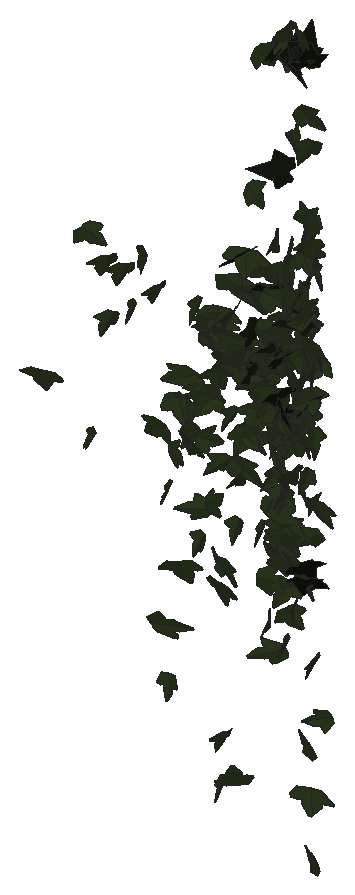
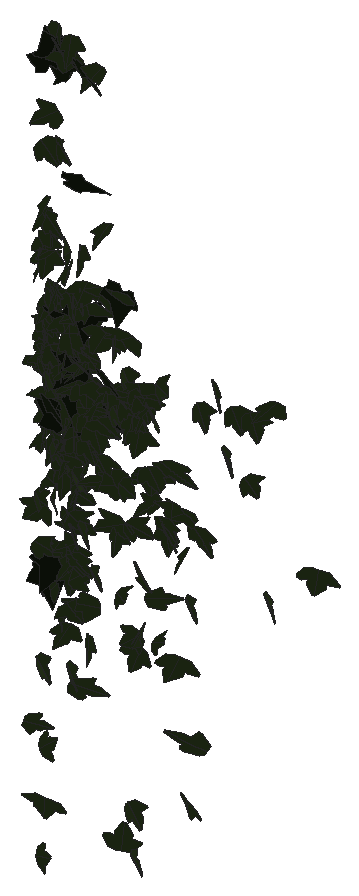
# SketchUp Ruby script. Lengths in millimetres.
U = 1.mm
M = Sketchup.active_model
def pt(a) = Geom::Point3d.new(a.map { |v| v * U })
def face(e, loops, mat)
  f = e.add_face(loops[0].map { |a| pt(a) })
  loops[1..].each { |l| e.add_face(l.map { |a| pt(a) }).erase! }
  f.material = f.back_material = mat if mat
  f
end
# faces: each face lists its corners as indices into pts; further lists are holes
def faces(e, pts, list, mat = nil) = list.each { |f| face(e, (f[0].is_a?(Array) ? f : [f]).map { |l| l.map { |i| pts[i] } }, mat) }
# xy, xz, yz: faces in a plane at the given z, y or x. An outline is a flat list of corners, or four numbers for a rectangle; further outlines are holes
def ring(l) = l.size == 4 ? [[l[0], l[1]], [l[2], l[1]], [l[2], l[3]], [l[0], l[3]]] : l.each_slice(2).to_a
def flat(e, list, mat, &to3) = list.each { |f| face(e, (f[0].is_a?(Array) ? f : [f]).map { |l| ring(l).map { |u, v| to3.(u, v) } }, mat) }
def xy(e, z, list, mat = nil) = flat(e, list, mat) { |x, y| [x, y, z] }
def xz(e, y, list, mat = nil) = flat(e, list, mat) { |x, z| [x, y, z] }
def yz(e, x, list, mat = nil) = flat(e, list, mat) { |y, z| [x, y, z] }
def lines(e, pts, list) = list.each { |a, b| e.add_line(pt(pts[a]), pt(pts[b])) }
# prism: a flat outline (further loops are holes) pulled along v
def prism(e, loops, v, mat = nil)
  f = face(e, loops, mat); d = Geom::Vector3d.new(v.map { |x| x * U })
  f.pushpull(f.normal.samedirection?(d) ? d.length : -d.length)
end
def box(e, o, s, mat = nil) = prism(e, [[o, [o[0] + s[0], o[1], o[2]], [o[0] + s[0], o[1] + s[1], o[2]], [o[0], o[1] + s[1], o[2]]]], [0, 0, s[2]], mat)
def at(x, y, z, deg = 0) = Geom::Transformation.translation(pt([x, y, z])) * Geom::Transformation.rotation(ORIGIN, Z_AXIS, deg.degrees)
def axes(o, x, y, z) = Geom::Transformation.new([*x, 0, *y, 0, *z, 0, *pt(o).to_a, 1])
def part(name) = M.definitions.add(name)
# library, detail: a bought-in or finely detailed component or shape, given as its bounding box
def library(name, o, s) = part(name).tap { |d| box(d.entities, o, s) }
def detail(e, o, s) = box(e.add_group.entities, o, s)
def put(e, d, t, mat = nil) = e.add_instance(d, t).tap { |i| i.material = mat if mat }
def group(e, t, mat = nil) = e.add_group.tap { |g| g.transformation = t; g.material = mat if mat }.entities
root = M.entities
M.materials.add("efeu1").color = [18, 25, 13]
M.materials.add("efeu2").color = [43, 57, 29]
c1 = part("ivyleaf_10")
p = [[0,12.8,-0.8],[-1.5,51.3,-10.9],[-4.9,51,-11.6],[-13.6,26.5,-7.3],[-13.2,15.9,-4.6],[-21.1,19.3,-7.2],
  [-29.5,16.3,-8.3],[-29.2,8.3,-6.2],[-19.7,-9.8,0.5],[-7.6,-13,4],[1,-12.2,5.8],[-0.4,51.1,-11.1],
  [-1.5,51.1,-10.9],[1,-12.4,5.9],[16.9,-12.4,3.5],[35.1,9.1,-5.1],[35,12.9,-6.1],[20.5,16.4,-4.9],
  [15.8,15,-3.8],[15.3,27.6,-7.1],[12.8,31.3,-7.8]]
faces(c1.entities,p,[[0,1,2,3,4,5,6,7,8,9,10],[11,12,0,13,14,15,16,17,18,19,20]],"efeu2")
c2 = part("ivyleaf_9")
p = [[39.1,54.8,31.7],[34.5,51.8,30.2],[-5.3,25.2,17.3],[-17.9,28.3,20.9],[-21.6,21.7,17],[-20.2,4.3,5.3],
  [-22.9,-0.3,2.5],[-17.1,-4,-0.6],[-2,-2.1,-1.2],[-0.7,-15.4,-10.1],[16.6,-22.3,-16.7],[21.1,-15.1,-12.5],
  [32.7,-10.7,-11],[46.1,-1.8,-6.6],[30.8,11.2,3.8]]
faces(c2.entities,p,[[0,1,2,3,4,5,6,7,8,9,10,11,12,13,14]],"efeu1")
put(root,c1,axes([243.8,1024.8,775],[-1.14378,-0.21353,-0.03623],[0.06369,0.01404,-0.63778],[0.40725,-0.6019,-0.00202]))
put(root,c1,axes([318.4,1039.9,1052.9],[-0.41994,-0.50459,-0.42857],[0.71436,0.27677,-0.51911],[1.03788,-0.39466,0.18389]))
put(root,c1,axes([342,1025,696.7],[0.38204,-0.58166,-0.17189],[-0.14186,0.15603,-0.61504],[1.1456,0.2133,-0.01884]))
put(root,c1,axes([360.7,1039,1016.2],[-0.43094,-0.65307,0.02889],[-0.01692,-0.02749,-0.69121],[1.24403,-0.22661,0.0006]))
put(root,c1,axes([361.3,1048.7,909],[-0.23851,-0.5727,0.31845],[0.11233,-0.33277,-0.57522],[1.24206,-0.07988,0.11318]))
put(root,c1,axes([397.1,1038.3,1014.2],[-0.38122,-0.64966,0.13016],[0.02244,-0.13945,-0.67789],[1.26081,-0.19395,0.05142]))
put(root,c1,axes([407.2,1046.4,941.3],[0.45731,-0.62845,-0.07217],[-0.01452,0.07432,-0.67255],[1.20385,0.23963,0.0193]))
put(root,c1,axes([435.8,1037.2,1047],[0.52125,-0.55892,-0.32588],[-0.13524,0.32574,-0.61842],[1.22389,0.27404,0.07045]))
put(root,c1,axes([462,1041.9,999.4],[-0.17968,-0.68576,-0.01445],[0.00325,0.01435,-0.69223],[1.30542,-0.09443,-0.00026]))
put(root,c1,axes([482,1020.7,764.2],[0.9589,-0.21043,-0.3824],[-0.4983,0.32157,-0.52193],[0.66465,0.54468,0.1604]))
put(root,c1,axes([483.5,1041.4,647.3],[0.34967,-0.60834,0.06607],[0.05066,-0.06098,-0.63543],[1.1635,0.18548,0.00781]))
put(root,c1,axes([478.2,1048.8,295.3],[0.89969,-0.38948,0.22707],[0.33701,-0.14216,-0.6125],[0.78909,0.50479,0.0027]))
put(root,c1,axes([468.8,1037.5,395.5],[-0.43167,-0.0979,0.62095],[1.06668,0.26745,0.24689],[-0.54178,0.60456,-0.00867]))
put(root,c1,axes([503.9,1027.4,724.5],[-0.31159,0.54731,0.35458],[-0.18791,0.34056,-0.57127],[-1.22682,-0.19117,-0.00256]))
put(root,c1,axes([492,1048.2,805.8],[0.88439,-0.12531,0.43496],[0.80746,-0.09668,-0.48112],[0.30026,0.62911,0.0127]))
put(root,c1,axes([505.1,1040.1,805],[1.20743,0.13863,0.1945],[0.34921,0.07053,-0.64877],[-0.29102,0.65981,0.02849]))
put(root,c1,axes([533.6,1032.4,868.9],[0.90647,-0.0279,-0.50428],[-0.95645,0.04266,-0.47702],[0.09546,0.69233,0.00907]))
put(root,c1,axes([518.9,1027.4,524.6],[-1.06041,-0.35067,-0.20841],[0.33868,0.10852,-0.65833],[0.69861,-0.58489,0.00281]))
put(root,c1,axes([530.8,1039,759.3],[0.63819,-0.53591,-0.09551],[-0.12462,0.07165,-0.63193],[1.02849,0.34122,-0.01731]))
put(root,c1,axes([537.1,1031,748.7],[-0.95721,0.27441,0.28094],[-0.45178,0.15124,-0.57268],[-0.59544,-0.55589,-0.01712]))
put(root,c1,axes([537.1,1037.9,771],[0.83249,-0.27794,-0.37958],[-0.47643,0.30133,-0.50912],[0.7581,0.49459,0.09687]))
put(root,c1,axes([536.8,1056.3,565.8],[-0.13218,-0.30835,0.55556],[0.40176,-0.53832,-0.27239],[1.14059,0.15389,0.16033]))
put(root,c1,axes([553.3,1042.8,631.3],[-0.04375,0.08652,0.64605],[-0.45722,-0.60207,0.07208],[1.15322,-0.23542,0.05309]))
put(root,c1,axes([549.1,1033.1,1005.5],[0.0982,-0.51268,0.47251],[0.34166,-0.44805,-0.50575],[1.28218,0.15865,0.09858]))
put(root,c1,axes([560.8,1039.7,852.4],[-0.72244,-0.50761,0.18659],[-0.08032,-0.19947,-0.6285],[1.02615,-0.37298,0.08217]))
put(root,c1,axes([553.9,1040.2,943],[0.8222,-0.52624,0.02536],[0.0078,0.03615,0.68035],[-1.00267,-0.43124,0.02609]))
put(root,c1,axes([568.7,1031,844.3],[-1.0269,-0.38209,-0.00867],[0.01608,0.00307,-0.66115],[0.7272,-0.53962,0.00238]))
put(root,c1,axes([572.4,1041.9,974],[-0.51232,-0.63261,0.04342],[0.08158,-0.06521,-0.68443],[1.20405,-0.26475,0.06485]))
put(root,c1,axes([577,1030.7,840.2],[0.57931,0.44445,-0.38843],[-0.55663,-0.26605,-0.53361],[-0.9758,0.41563,0.07379]))
put(root,c1,axes([573.5,1035.5,953.4],[-0.23927,0.56866,0.35734],[-0.17884,0.34508,-0.58221],[-1.26565,-0.15627,0.01471]))
put(root,c1,axes([577.8,1041.3,986.5],[-0.68469,-0.58708,0.07461],[0.05214,-0.10375,-0.68421],[1.12511,-0.35246,0.07711]))
put(root,c1,axes([569.4,1039.7,647.3],[0.66681,-0.44946,-0.33138],[0.40455,-0.25441,0.5698],[-0.98277,-0.40969,0.00971]))
put(root,c1,axes([577.9,1010.2,780.2],[0.09037,0.2806,0.64845],[0.00055,0.6499,-0.28125],[-1.34471,0.01912,0.04346]))
put(root,c1,axes([573.5,1042.2,974.9],[0.99148,0.43636,0.1171],[0.17152,0.07478,-0.67956],[-0.84259,0.52869,-0.00054]))
put(root,c1,axes([581.8,1041.1,996.8],[1.02653,0.42733,-0.09746],[-0.24998,0.01015,-0.68241],[-0.79584,0.54801,0.08864]))
put(root,c1,axes([594.4,1035.1,541.1],[-0.49843,0.61671,-0.02893],[-0.05656,0.0188,0.66972],[1.17365,0.26281,0.01999]))
put(root,c1,axes([594.1,1028.1,898.6],[-0.67247,-0.55847,-0.13766],[0.25347,0.07773,-0.65719],[1.06494,-0.37115,0.06949]))
put(root,c1,axes([591.5,1041.5,154.7],[0.53797,-0.53181,0.27789],[0.23475,-0.24912,-0.60222],[1.11759,0.30832,-0.00727]))
put(root,c1,axes([598.7,1039.8,242.6],[-0.10217,-0.66898,0.10962],[-0.01804,-0.10921,-0.67113],[1.29005,-0.05451,-0.00071]))
put(root,c1,axes([602.4,1034.2,739.4],[-0.22571,-0.41896,0.51867],[-0.18294,-0.51056,-0.4344],[1.25569,-0.14969,0.02994]))
put(root,c1,axes([596.7,1027.8,515.1],[-1.1334,0.31842,-0.00472],[0.00764,-0.0025,-0.67531],[-0.60604,-0.59554,0.00031]))
put(root,c1,axes([591.6,1039.6,550.2],[-0.81529,0.39711,-0.32232],[0.44589,-0.22138,-0.58412],[-0.86528,-0.48825,0.00269]))
put(root,c1,axes([603.5,1054.5,818.3],[0.01043,-0.48929,0.44481],[0.17887,-0.43973,-0.48486],[1.24572,0.06724,0.0659]))
put(root,c1,axes([607.9,1028.7,920.2],[-0.39697,-0.59069,-0.26106],[0.21059,0.23759,-0.626],[1.21093,-0.23496,0.02328]))
put(root,c1,axes([611.6,1037.5,1005.4],[0.03361,-0.69736,0.01255],[-0.00367,-0.0126,-0.69758],[1.32743,0.01762,-0.00225]))
put(root,c1,axes([611.8,1029.8,971.8],[-1.35976,0.1047,-0.07512],[0.14071,-0.01356,-0.72209],[-0.20087,-0.71827,0.00268]))
put(root,c1,axes([611.2,1025,928.9],[-1.1707,0.28049,-0.09416],[0.16021,-0.04234,-0.67604],[-0.53983,-0.62085,0.00356]))
put(root,c1,axes([612.6,1052.7,621.4],[-0.1487,-0.47329,0.43932],[0.39991,-0.43708,-0.4335],[1.16213,0.08984,0.20539]))
put(root,c1,axes([635,1027,957.9],[0.76154,-0.07642,-0.55362],[-1.03185,0.11214,-0.40734],[0.2581,0.67381,0.005]))
put(root,c1,axes([623.3,1035.4,167.6],[-0.78033,-0.5067,-0.17803],[-0.21021,-0.13963,0.6518],[-1.00029,0.42462,0.0019]))
put(root,c1,axes([628.1,1040.7,935.7],[-0.07877,-0.67113,0.12702],[-0.02779,-0.12635,-0.67237],[1.29967,-0.04338,-0.00668]))
put(root,c1,axes([629.6,1036,950.6],[-1.3052,-0.04189,-0.0047],[0.00893,0.00025,-0.68707],[0.07972,-0.68581,0.00004]))
put(root,c1,axes([642.2,1020.5,930.4],[0.35996,-0.11662,-0.73562],[-0.83909,0.26101,-0.31724],[0.34873,0.74838,-0.00399]))
put(root,c1,axes([628.9,1038,718.7],[-0.19403,-0.54483,-0.38034],[0.10211,0.37679,-0.55412],[1.26046,-0.11439,-0.01366]))
put(root,c1,axes([615.5,1033.3,1068.9],[-1.0356,-0.05293,-0.45602],[0.85745,-0.19739,-0.51468],[-0.16781,-0.68196,0.18437]))
put(root,c1,axes([639,1031.5,1056.1],[0.15534,-0.39829,-0.58429],[-0.08218,0.58426,-0.40431],[1.34329,0.0818,0.04283]))
put(root,c2,axes([641.8,1010.9,1129],[0.20859,0.77501,0.18738],[-0.07646,0.20411,-0.78701],[-0.96974,0.15061,0.10236]))
put(root,c2,axes([658.2,1028.6,917.1],[-0.23068,0.34056,0.67745],[-0.39286,0.59603,-0.38951],[-0.83748,-0.3734,-0.00388]))
put(root,c1,axes([622,1039.5,738.4],[0.85401,0.01675,0.51547],[0.93499,0.1941,-0.43396],[-0.29877,0.65528,0.11537]))
put(root,c2,axes([657.7,1037.8,989],[-0.69618,0.49708,0.06067],[-0.06079,0.03517,-0.75676],[-0.60791,-0.57278,0.00619]))
put(root,c1,axes([647.6,1023.4,955.4],[-0.32606,-0.67874,-0.19466],[0.18094,0.17631,-0.69843],[1.33162,-0.19015,0.04724]))
put(root,c1,axes([651.5,1026.8,808.7],[0.69087,0.49212,-0.25041],[-0.34856,-0.0458,-0.7361],[-0.57645,0.61749,0.14497]))
put(root,c1,axes([655.9,1045.7,909.6],[0.84485,0.35841,-0.37874],[-0.58651,-0.22092,-0.57025],[-0.80056,0.54009,0.01808]))
put(root,c1,axes([640.8,1026.9,962.5],[-0.58218,-0.44364,-0.48768],[0.69405,0.33402,-0.5326],[1.04531,-0.46887,0.08202]))
put(root,c1,axes([649.3,1025.9,1131.2],[1.28998,0.2556,0.04802],[0.08082,0.02348,-0.72435],[-0.48832,0.67909,0.00697]))
put(root,c1,axes([636.8,1042.4,802.7],[0.67441,-0.19668,0.54592],[1.06191,-0.06016,-0.38385],[0.30326,0.64806,0.13004]))
put(root,c1,axes([658.8,1033.4,1060.6],[-1.31735,-0.07129,-0.16335],[0.30841,0.02101,-0.69583],[0.14123,-0.71088,-0.00419]))
put(root,c1,axes([666.9,1045.9,890.9],[-0.70261,-0.566,0.05797],[-0.05198,-0.05139,-0.67573],[1.08159,-0.37015,0.00518]))
put(root,c1,axes([658.2,1031.1,1247.8],[0.03103,0.66229,0.34031],[0.03271,0.33947,-0.66267],[-0.90783,0.03487,-0.01224]))
put(root,c1,axes([665.7,1039.8,844.1],[1.29378,-0.07946,-0.10379],[-0.19291,0.02668,-0.68427],[0.1571,0.68715,0.01456]))
put(root,c1,axes([657.6,1029.6,800.5],[0.02303,0.03073,0.69844],[0.32224,0.67762,-0.03275],[-1.29094,0.16969,0.00429]))
put(root,c1,axes([666.9,1046.9,637.6],[0.47389,-0.57995,0.20296],[0.16603,-0.1834,-0.6311],[1.15755,0.26373,0.00743]))
put(root,c1,axes([669.5,1042.8,934.2],[-0.15364,0.68418,-0.04311],[0.00361,-0.04318,-0.68892],[-1.30471,-0.08069,0.00317]))
put(root,c1,axes([691.9,1042.3,923.5],[-0.01719,0.02864,-0.69702],[-0.85042,0.02692,0.0152],[0.03358,0.69664,0.02807]))
put(root,c1,axes([680.8,1045.8,864.1],[-0.54027,-0.59707,0.11599],[0.01712,-0.1321,-0.65803],[1.15746,-0.27674,0.06387]))
put(root,c1,axes([683.1,1045.7,904.2],[-0.3846,-0.64927,-0.03225],[0.02682,0.02939,-0.67998],[1.23693,-0.20252,0.00472]))
put(root,c1,axes([701.6,1044.5,425.1],[-0.36828,-0.12279,0.63408],[-0.59973,-0.55985,-0.20458],[1.07297,-0.35507,0.10329]))
put(root,c1,axes([692.7,1040.4,952.4],[-0.71318,-0.5705,0.12323],[-0.0061,-0.14442,-0.67838],[1.1108,-0.36708,0.07539]))
put(root,c1,axes([685.9,1017.2,1510.8],[0.22259,0.50471,0.55421],[-0.00574,0.57115,-0.51859],[-0.91448,0.11926,0.13815]))
put(root,c1,axes([696,1048.3,860.3],[-0.80007,-0.50018,0.15074],[-0.06512,-0.16671,-0.64858],[0.99209,-0.41431,0.07899]))
put(root,c1,axes([695.9,1026.6,1086.6],[-0.76815,-0.58965,0.08348],[-0.02617,-0.09159,-0.71343],[1.13311,-0.40185,0.04011]))
put(root,c1,axes([689.4,1037.2,824.8],[-0.27165,0.59603,-0.26917],[0.00542,-0.27494,-0.61031],[-1.24466,-0.13128,0.05609]))
put(root,c1,axes([700.4,1034,897.6],[-0.51315,-0.53898,0.30992],[-0.12433,-0.31138,-0.59835],[1.17673,-0.26794,0.07193]))
put(root,c1,axes([694.3,1044.7,706],[0.41316,-0.5912,0.09438],[0.06737,-0.08754,-0.62979],[1.13743,0.21993,0.00302]))
put(root,c1,axes([695,1040,967.8],[-0.8957,-0.51286,-0.07817],[0.37172,-0.07739,-0.6682],[0.9147,-0.47076,0.195]))
put(root,c1,axes([691.8,1040.4,994],[0.52514,0.61919,0.13479],[0.08915,0.11336,-0.75409],[-0.76794,0.43658,0.00463]))
put(root,c1,axes([702.7,1016.2,492.5],[0.12999,-0.55823,-0.51413],[-0.1094,0.50628,-0.56828],[0.91939,0.13917,0.00507]))
put(root,c2,axes([700.9,1021.1,1089.9],[0.58187,0.59197,-0.27746],[-0.21923,-0.21151,-0.76016],[-0.76687,0.50962,0.0068]))
put(root,c1,axes([699.5,1051.2,802.1],[0.32165,-0.58916,0.2344],[0.08958,-0.23026,-0.61268],[1.20344,0.17461,-0.01704]))
put(root,c1,axes([682.8,1028.4,1005.2],[-0.03419,-0.06275,-0.71995],[0.80169,-0.30207,0.00075],[-0.36694,-0.65412,0.06872]))
put(root,c1,axes([707,1043.1,650],[0.67254,-0.0916,-0.40363],[-0.48842,0.05261,-0.55871],[0.12815,0.68121,-0.01112]))
put(root,c2,axes([710.8,1032.5,1523.5],[-0.7193,0.46986,-0.10387],[0.08585,-0.07832,-0.75372],[-0.58076,-0.59353,0.01723]))
put(root,c1,axes([700.4,1037.4,1005.6],[0.89302,-0.2266,-0.07968],[-0.08795,0.03653,-0.76613],[0.27953,0.7354,0.0135]))
put(root,c2,axes([716.8,1034.3,996.3],[-0.82568,0.36867,0.02666],[-0.07152,-0.05214,-0.76715],[-0.44525,-0.6753,0.07379]))
put(root,c1,axes([689.9,1040.4,964.6],[-0.8136,-0.20493,-0.51144],[0.89647,0.19988,-0.47381],[0.54397,-0.6359,0.01589]))
put(root,c1,axes([703.8,1037.9,843.9],[0.46941,-0.66296,0.06145],[0.06917,-0.03809,-0.76594],[0.80933,0.38778,0.02982]))
put(root,c1,axes([702.2,1025.8,1123.8],[-0.78422,-0.53674,-0.26792],[0.38084,0.18344,-0.67526],[1.07633,-0.45598,0.04372]))
put(root,c1,axes([702.2,1036.8,993.4],[-0.40142,0.66772,0.08289],[-0.0128,0.08477,-0.69999],[-1.2805,-0.21017,-0.01899]))
put(root,c1,axes([716.8,1026,1110.1],[-0.32102,0.25906,0.61267],[-0.65694,0.30386,-0.35975],[-0.47645,-0.59352,0.08324]))
put(root,c1,axes([712.5,1031,757.7],[0.29192,0.48706,-0.49016],[-0.51591,-0.41944,-0.50161],[-1.2097,0.29641,0.09564]))
put(root,c1,axes([710.6,1039.5,756.8],[-0.28102,0.70236,0.12245],[0.03611,-0.11915,0.73912],[0.86906,0.23207,0.00888]))
put(root,c1,axes([691.1,1023.7,561.9],[-0.04262,-0.00707,-0.79493],[0.9628,0.09553,-0.03553],[0.11681,-0.78994,0.00281]))
put(root,c1,axes([714.7,1041,718.8],[-0.52329,-0.45174,0.43415],[-0.02426,-0.46998,-0.4971],[1.19218,-0.20785,0.18044]))
put(root,c1,axes([724,1028.6,601.6],[-0.62273,0.08714,-0.52601],[-0.64288,0.02846,0.51607],[0.09908,0.7324,0.04253]))
put(root,c2,axes([729.1,1029.9,1306.1],[-0.66681,0.07563,0.53038],[-0.64562,0.04185,-0.55132],[-0.10185,-0.76045,0.0224]))
put(root,c1,axes([714.7,1030.8,872.5],[0.08711,-0.50795,-0.43559],[-0.05731,0.43317,-0.51284],[0.81434,0.08482,0.0105]))
put(root,c1,axes([713.9,1021,1183],[0.13378,-0.64335,-0.36683],[0.14809,0.37286,-0.63901],[1.40168,0.02201,0.10252]))
put(root,c2,axes([704.9,1037.1,993.5],[0.91214,0.16727,-0.0198],[-0.02428,-0.00173,-0.76614],[-0.20405,0.74792,0.00265]))
put(root,c1,axes([716.9,1044.9,449.5],[0.28801,-0.61984,-0.00619],[-0.00331,0.00594,-0.63804],[1.17973,0.15134,-0.00028]))
put(root,c1,axes([726.4,1027.7,646.3],[-0.68936,-0.28517,0.36611],[-0.40099,-0.16131,-0.63292],[0.39969,-0.65368,-0.00353]))
put(root,c1,axes([716.7,1043.1,703.7],[0.57547,-0.57647,-0.03784],[-0.0287,0.02965,-0.74486],[0.70422,0.47228,0.00057]))
put(root,c1,axes([712.5,1030.5,865.9],[-0.53763,-0.5992,-0.21261],[0.41678,-0.00498,-0.69406],[0.6542,-0.48926,0.26745]))
put(root,c1,axes([703,1020.6,1077.2],[0.31986,0.23896,0.72676],[0.58533,0.54704,-0.35295],[-0.72699,0.54559,0.03558]))
put(root,c1,axes([712.2,1029.3,818],[-0.12776,-0.35691,0.59645],[0.18613,0.57666,0.37186],[-0.82732,0.18486,-0.00844]))
put(root,c1,axes([728.6,1034.9,1101.1],[-0.63024,0.21566,0.42487],[-0.49711,0.12486,-0.55881],[-0.30131,-0.6571,0.03326]))
put(root,c2,axes([724.9,1015,910.7],[0.15277,0.77737,-0.09638],[-0.0223,-0.09468,-0.78738],[-0.95539,0.12651,0.00297]))
put(root,c1,axes([729.4,1041.4,969.4],[-0.07299,-0.06421,-0.74602],[-0.59392,-0.5653,0.08769],[-0.69409,0.49047,0.00341]))
put(root,c1,axes([718.8,1029,756.6],[-0.49296,0.55374,-0.1092],[0.07966,-0.08754,-0.68549],[-0.68395,-0.40931,-0.00113]))
put(root,c1,axes([726,1031.7,1025.7],[-0.52852,-0.65594,-0.01572],[0.01204,0.01439,-0.71231],[1.24869,-0.27777,0.00021]))
put(root,c1,axes([724.2,1037.7,554.7],[0.54774,0.50651,-0.3677],[-0.33353,-0.24837,-0.67594],[-0.68691,0.52449,0.035]))
put(root,c1,axes([727.4,1030.2,795.8],[0.32256,-0.10421,0.57448],[-0.44798,0.46062,0.25255],[-0.55379,-0.43331,0.13031]))
put(root,c1,axes([724.2,1034.3,1557.6],[-0.2112,-0.68298,-0.32534],[0.08714,0.3175,-0.70453],[0.91882,-0.1871,-0.00797]))
put(root,c1,axes([724.3,1037.2,721],[0.03684,0.25247,-0.67775],[-0.13623,-0.66857,-0.25403],[-0.87178,0.11515,0.01106]))
put(root,c1,axes([721.6,1041.2,975.5],[0.21343,0.70188,0.01688],[0.00105,0.01718,-0.72334],[-0.85654,0.17491,0.00332]))
put(root,c1,axes([733.1,1027.4,1006.9],[-0.74827,-0.16436,0.25994],[-0.29381,-0.104,-0.63399],[0.23335,-0.65798,0.03527]))
put(root,c1,axes([727.7,1027.1,608.5],[-0.69981,-0.34446,-0.03193],[0.03329,0.01659,-0.6691],[0.42073,-0.57427,-0.00018]))
put(root,c1,axes([725.2,1032.1,817],[-0.02904,0.49786,0.49867],[-0.09926,0.49367,-0.49676],[-0.85392,-0.07431,0.04078]))
put(root,c1,axes([728.4,1031,883.2],[-0.51881,0.54581,0.3087],[-0.21301,0.28886,-0.60955],[-1.17425,-0.29355,-0.02582]))
put(root,c2,axes([709.9,1030.1,882],[0.17644,-0.00831,-0.76614],[0.93263,-0.05097,0.14486],[-0.06298,-0.77801,-0.00131]))
put(root,c1,axes([735.8,1036.8,815.3],[-0.70629,-0.30647,0.36606],[-0.28176,-0.32377,-0.63632],[0.50975,-0.60359,0.15547]))
put(root,c1,axes([732.3,1016.2,720.4],[0.14211,-0.36935,-0.6145],[-0.07442,0.61481,-0.37429],[1.36249,0.0721,0.04365]))
put(root,c1,axes([727.4,1032.1,662.1],[0.03348,-0.07316,0.66296],[-0.07024,0.66079,0.0753],[-0.81069,-0.06027,0.02086]))
put(root,c1,axes([726.7,1029.6,631.1],[-0.00802,0.49727,0.53231],[-0.03442,0.53176,-0.4971],[-0.88804,-0.0251,0.01446]))
put(root,c1,axes([714.6,1020.8,689.4],[1.20783,-0.03986,-0.32095],[0.6132,0.0167,0.63503],[-0.05331,-0.71097,0.03291]))
put(root,c1,axes([737.4,1034.9,967.9],[-0.7694,-0.52725,0.21041],[-0.11852,-0.21556,-0.65981],[1.0739,-0.40154,0.07793]))
put(root,c2,axes([719.9,1015.2,961.5],[0.28621,0.7189,-0.07508],[0.02113,0.07332,0.75618],[0.88158,-0.23515,0.00625]))
put(root,c1,axes([747.7,1035.5,1364],[-0.09247,0.14577,0.74173],[-0.85941,0.25678,-0.12244],[-0.33452,-0.69998,0.10955]))
put(root,c1,axes([739.1,1022.5,1048],[-0.84823,-0.32853,0.09744],[-0.11551,-0.02766,-0.76883],[0.40179,-0.70152,-0.01532]))
put(root,c1,axes([741.8,1022.5,1093.6],[-0.86818,0.2824,0.22154],[-0.3388,-0.12153,-0.73712],[-0.27742,-0.73534,0.2069]))
put(root,c1,axes([731,1034.4,511.6],[-0.52515,-0.48124,-0.35068],[0.40195,0.16796,-0.6349],[0.60513,-0.5292,0.1174]))
put(root,c2,axes([747.9,1023.5,1542.3],[-0.64856,0.55983,-0.11159],[0.02991,-0.12995,-0.76875],[-0.69579,-0.52742,0.07097]))
put(root,c1,axes([737.3,1042.3,911.3],[0.68101,-0.54445,-0.20408],[0.03161,0.2491,-0.63544],[1.10615,0.32808,0.1438]))
put(root,c1,axes([734.8,1035,1528.3],[0.85133,0.33472,-0.03971],[-0.08132,0.04755,-0.77062],[-0.4031,0.69732,0.07161]))
put(root,c1,axes([736.2,1029.8,987.7],[0.12735,-0.6186,-0.31639],[0.2196,0.32334,-0.60777],[1.30401,0.00596,0.13325]))
put(root,c1,axes([741,1021.5,955.7],[-0.76398,0.371,0.08656],[-0.09045,0.04468,-0.72787],[-0.45589,-0.63059,-0.00065]))
put(root,c2,axes([753.5,1024.1,1538.8],[-0.63639,0.58354,0.14992],[-0.1472,0.09311,-0.78222],[-0.72014,-0.5347,0.0274]))
put(root,c1,axes([737.1,1025.5,1145.6],[-0.11451,0.71736,-0.13127],[0.02669,-0.12953,-0.72346],[-0.88931,-0.09626,-0.00481]))
put(root,c1,axes([747.2,1013.4,1164.2],[0.28561,-0.2473,0.67716],[-0.51161,0.53241,0.33941],[-0.71539,-0.47948,0.02762]))
put(root,c1,axes([743.8,1046,835.4],[-0.02604,-0.66531,0.04219],[0.00615,-0.04226,-0.66543],[1.26874,-0.01345,0.00409]))
put(root,c1,axes([739.5,1035.4,1060],[0.30915,0.66378,-0.21334],[-0.09053,-0.20003,-0.7105],[-0.84577,0.26404,-0.00193]))
put(root,c1,axes([739.2,1035.8,841.2],[-0.13219,0.66905,-0.14828],[0.03125,-0.14606,-0.67777],[-0.83547,-0.11133,-0.00189]))
put(root,c1,axes([756.5,1036.3,839.4],[-0.54719,0.11191,0.53572],[-0.64971,0.07038,-0.46056],[-0.15387,-0.69513,0.03962]))
put(root,c2,axes([727.6,1034.9,1502.4],[0.35057,-0.59697,0.37739],[0.38658,-0.25515,-0.64488],[0.77005,0.39987,0.15193]))
put(root,c1,axes([747.5,1022.8,773.8],[-0.32888,-0.62468,-0.28309],[0.12545,0.27546,-0.64808],[1.29924,-0.18473,-0.00908]))
put(root,c1,axes([742,1035,520.2],[0.05137,-0.21788,-0.6056],[0.10824,-0.59914,0.22172],[-0.7777,-0.09778,-0.00915]))
put(root,c1,axes([732.6,1041.7,653.9],[-0.24252,-0.0151,-0.63074],[0.75179,-0.14657,-0.1907],[-0.16518,-0.64488,0.05811]))
put(root,c1,axes([765.6,1039.9,1230.5],[-0.38287,0.04141,0.63783],[-0.77377,0.06795,-0.31647],[-0.09672,-0.7076,0.00693]))
put(root,c1,axes([748.8,1027.8,876.6],[-0.78251,0.24795,-0.1796],[0.19604,-0.08226,-0.68742],[-0.31794,-0.66097,0.01818]))
put(root,c1,axes([749.6,1056.5,1093.9],[-0.01526,-0.23978,-0.66077],[0.00242,-0.66088,0.23978],[-0.85757,0.0024,0.01243]))
put(root,c1,axes([757.5,1036.6,997.2],[-0.53991,-0.61148,0.2043],[-0.00418,-0.22229,-0.66836],[1.227,-0.26982,0.08762]))
put(root,c1,axes([739.9,1054.9,742.9],[0.18952,-0.19788,0.61403],[0.78807,-0.45682,-0.21437],[0.9415,0.42221,0.05584]))
put(root,c2,axes([772.5,1030.1,1056.2],[-0.82594,0.07178,0.336],[-0.41188,-0.00112,-0.68],[-0.07784,-0.75579,0.03292]))
put(root,c1,axes([756.1,1039.9,830.9],[-0.6629,0.4269,-0.01992],[0.02217,-0.00911,-0.69099],[-0.52091,-0.54365,-0.00406]))
put(root,c1,axes([758.6,1028.2,1564.6],[-0.75983,0.48346,0.04788],[-0.09367,-0.02108,-0.78586],[-0.58526,-0.62429,0.06362]))
put(root,c1,axes([774.2,1022.1,1097.2],[-0.28113,0.16344,0.66486],[-0.82626,0.04838,-0.24662],[-0.12239,-0.70199,0.1378]))
put(root,c2,axes([746.5,1029.3,878.4],[0.54995,0.64029,-0.06184],[0.01034,0.06959,0.78236],[0.78472,-0.44965,0.03302]))
put(root,c1,axes([760.8,1026,1100.3],[0.04092,-0.56387,-0.46352],[0.14603,0.46289,-0.55955],[1.38151,-0.03222,0.07288]))
put(root,c2,axes([772.5,1028.7,904.1],[-0.57563,0.62464,-0.04782],[0.03119,-0.04062,-0.7828],[-0.76365,-0.47251,0.00407]))
put(root,c1,axes([771.9,1051.7,655.2],[-0.28119,-0.28788,0.54307],[-0.39763,-0.4345,-0.36865],[0.63577,-0.39907,0.00963]))
put(root,c1,axes([769.1,1043.4,1361.3],[-0.33914,-0.59908,0.34965],[-0.16604,-0.32226,-0.66035],[0.82981,-0.30932,0.01077]))
put(root,c1,axes([758,1039.5,962.2],[0.53241,-0.51554,0.32677],[0.30702,-0.214,-0.6737],[0.67842,0.50143,0.04844]))
put(root,c2,axes([764.7,1032.7,1525.9],[-0.48843,-0.31504,0.58593],[0.5613,0.36282,0.50944],[-0.58622,0.60988,-0.0004]))
put(root,c1,axes([767,1032.9,949.2],[0.08976,-0.68441,0.09525],[0.04787,-0.09371,-0.68579],[1.31426,0.05016,0.01848]))
put(root,c1,axes([766.6,1042.4,1166.5],[-0.64237,-0.46657,-0.10247],[0.09352,0.068,-0.70351],[0.57523,-0.53209,-0.00006]))
put(root,c1,axes([775.5,1024.7,1095.3],[-0.14462,0.3022,0.62893],[-0.6065,0.41107,-0.29122],[-0.59735,-0.49053,0.14342]))
put(root,c1,axes([758.8,1034.7,579.1],[-0.55248,0.32436,-0.36513],[0.37385,-0.19903,-0.55685],[-0.46396,-0.54661,-0.01391]))
put(root,c1,axes([766.2,1039.4,770.3],[0.06299,0.47306,-0.43575],[-0.11077,-0.42741,-0.47477],[-0.7768,0.09931,0.03237]))
put(root,c1,axes([763.1,1031.8,1164.7],[0.23469,0.64879,0.20005],[0.0658,0.19266,-0.67671],[-0.82568,0.19976,0.00293]))
put(root,c2,axes([763.5,1037.5,1506.9],[0.61329,0.42833,0.39648],[-0.40209,-0.22353,0.65937],[0.58768,-0.59994,0.03739]))
put(root,c1,axes([768.9,1032.5,880.8],[-0.55424,-0.59704,-0.08792],[0.18754,-0.00807,-0.73951],[0.71196,-0.46265,0.12635]))
put(root,c1,axes([774.5,1031.6,1047.1],[-0.54251,-0.6104,0.24274],[-0.01312,-0.26182,-0.66646],[1.25014,-0.26764,0.09835]))
put(root,c2,axes([769.5,1014.3,615.5],[0.54963,0.6646,0.04239],[0.03329,0.03271,-0.80289],[-0.81177,0.45132,-0.00423]))
put(root,c1,axes([773,1037.3,1186.9],[-0.52566,-0.5345,-0.05392],[0.04507,0.03947,-0.68653],[0.65385,-0.43243,0.00398]))
put(root,c1,axes([778.9,1032.2,911.1],[0.2263,0.1526,-0.62744],[-0.55365,-0.43361,-0.23962],[-0.56044,0.48997,-0.01664]))
put(root,c1,axes([768.3,1031.7,1188.4],[-0.02358,-0.70925,-0.29727],[-0.01352,-0.29708,0.70951],[-0.93812,0.02211,-0.00276]))
put(root,c1,axes([783.3,1012.8,987.4],[-0.064,0.06508,-0.70544],[-0.51414,0.56573,0.08353],[0.69473,0.42467,-0.00317]))
put(root,c2,axes([778,1018.7,591.7],[0.46058,0.58895,-0.35695],[-0.36254,-0.22791,-0.69033],[-0.75795,0.4669,0.11329]))
put(root,c1,axes([777.4,1027.7,1067.4],[-0.29357,-0.69934,0.08715],[-0.03771,-0.08488,-0.71615],[1.34074,-0.15552,-0.00106]))
put(root,c1,axes([785,1024.4,280.1],[-0.50517,0.3247,-0.50915],[-0.51983,0.28038,0.52533],[0.52207,0.59337,0.03039]))
put(root,c1,axes([770.5,1041.1,983.9],[0.61782,0.45036,-0.05576],[-0.05061,-0.03726,-0.6777],[-0.55132,0.50811,-0.00027]))
put(root,c1,axes([758.5,1035.9,1418.9],[0.56049,0.00439,0.59474],[0.61705,0.39251,-0.3936],[-0.38176,0.64087,0.23699]))
put(root,c1,axes([769,1021,986.4],[0.29062,0.38494,0.58832],[0.10104,0.60148,-0.42709],[-0.85177,0.20269,0.15007]))
put(root,c1,axes([774.5,1029.6,1075.7],[-0.16979,-0.49336,-0.45798],[0.14227,0.44292,-0.51257],[0.80884,-0.18147,-0.00598]))
put(root,c1,axes([780.9,1025.1,1016.6],[-0.87798,0.08511,0.17442],[-0.21538,-0.00885,-0.7241],[-0.09835,-0.74044,0.0287]))
put(root,c1,axes([771.1,1023,1046.9],[0.69052,0.39545,-0.18804],[0.18508,0.11118,0.69045],[0.50113,-0.58596,0.0041]))
put(root,c1,axes([776,1038,1231],[0.08582,0.59572,-0.35334],[-0.15257,-0.33839,-0.59543],[-0.83112,0.12364,0.07282]))
put(root,c1,axes([778.1,1041.4,438.5],[0.24969,-0.67833,0.12845],[0.03535,-0.12724,-0.69088],[1.31347,0.13238,-0.00582]))
put(root,c1,axes([769.9,1039.9,195.1],[1.28108,0.07528,0.08797],[0.16546,0.01412,-0.6773],[-0.14555,0.6787,0.00433]))
put(root,c1,axes([773.6,1034.5,919.4],[0.47817,0.58267,0.14037],[0.01617,0.15926,-0.69806],[-0.73101,0.38466,0.07638]))
put(root,c1,axes([775.1,1042.9,977.6],[0.07375,-0.39403,0.56988],[0.29838,-0.52308,-0.38761],[0.79084,0.2341,0.0931]))
put(root,c1,axes([776.9,1039.9,843.7],[-0.01607,0.74417,-0.12889],[-0.03322,-0.12929,-0.74372],[-0.92081,-0.00832,0.02908]))
put(root,c1,axes([784.3,1030.2,1172.3],[0.20089,0.00962,-0.6977],[-0.15476,0.70533,-0.02021],[0.83709,0.12809,0.1637]))
put(root,c1,axes([787.3,1021.9,956.4],[-0.28402,0.57275,0.37531],[-0.44623,0.23111,-0.57957],[-0.70625,-0.37636,0.21526]))
put(root,c1,axes([792.1,1050.6,333.8],[0.21436,0.08984,-0.6067],[-0.69343,-0.21326,-0.19619],[-0.28112,0.59454,0.02131]))
put(root,c1,axes([781.9,1041.6,731.8],[0.12137,-0.60765,0.19177],[0.09928,-0.1871,-0.6102],[1.20863,0.07639,0.03087]))
put(root,c1,axes([780.8,1039.3,997],[-0.60331,0.54874,-0.01723],[0.01285,-0.0137,-0.73869],[-0.66967,-0.49462,0.00135]))
put(root,c1,axes([795.2,1022,80.6],[-0.23969,0.23082,-0.65359],[-0.5552,0.46947,0.30259],[0.63786,0.49536,0.01778]))
put(root,c1,axes([785.7,1018.6,1244.4],[-0.21433,0.58332,0.39693],[-0.16257,0.37426,-0.60898],[-0.84529,-0.21988,0.01648]))
put(root,c1,axes([789.5,1027.5,1046.3],[0.37653,-0.60344,-0.33031],[-0.12785,0.32511,-0.63417],[1.303,0.20628,0.03322]))
put(root,c1,axes([787.6,1043.5,975],[0.74999,0.08364,-0.24112],[-0.29189,-0.03001,-0.62041],[-0.10837,0.65966,0.00235]))
put(root,c1,axes([777.5,1045,716.2],[-1.04866,0.25416,-0.27255],[0.44825,-0.13951,-0.60625],[-0.54965,-0.59868,0.02557]))
put(root,c1,axes([783.8,1036.7,1146],[-0.35123,0.61659,0.02274],[-0.00898,0.02166,-0.68049],[-0.7527,-0.28798,-0.00249]))
